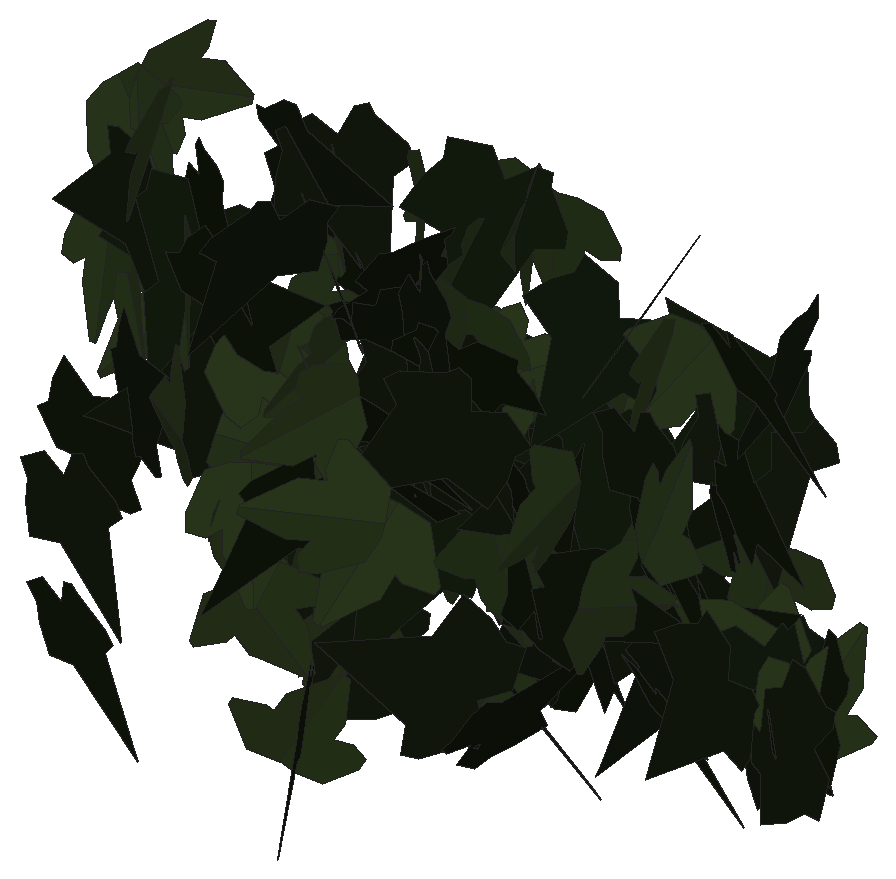
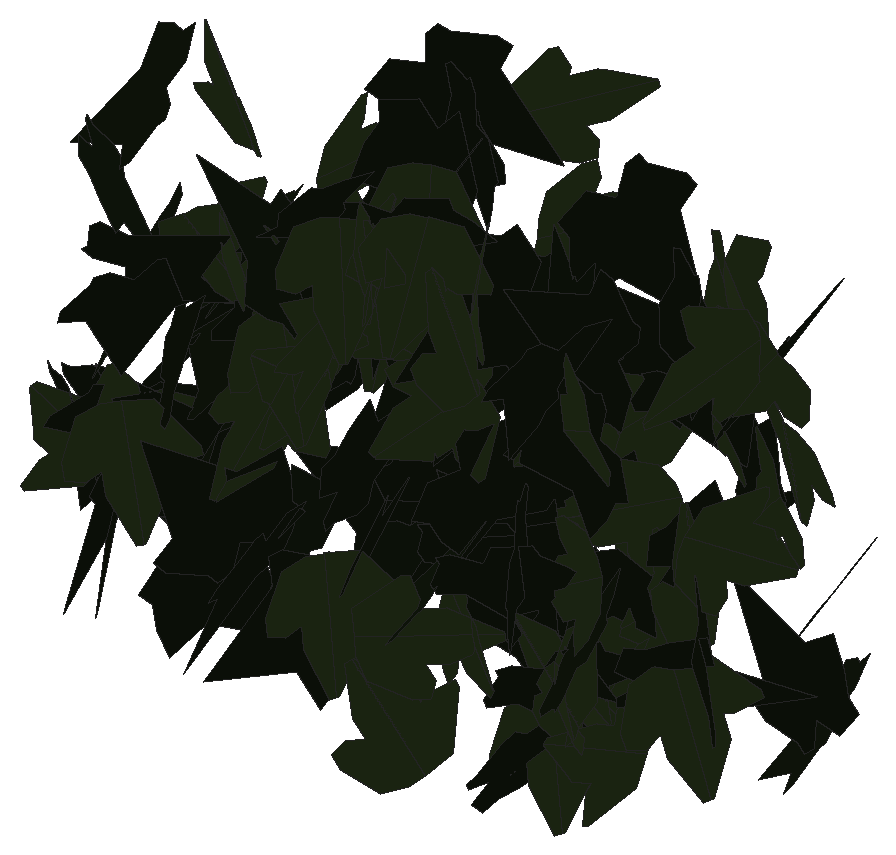
# SketchUp Ruby script. Lengths in inches.
U = 1.inch
M = Sketchup.active_model
def pt(a) = Geom::Point3d.new(a.map { |v| v * U })
def face(e, loops, mat)
  f = e.add_face(loops[0].map { |a| pt(a) })
  loops[1..].each { |l| e.add_face(l.map { |a| pt(a) }).erase! }
  f.material = f.back_material = mat if mat
  f
end
# faces: each face lists its corners as indices into pts; further lists are holes
def faces(e, pts, list, mat = nil) = list.each { |f| face(e, (f[0].is_a?(Array) ? f : [f]).map { |l| l.map { |i| pts[i] } }, mat) }
# xy, xz, yz: faces in a plane at the given z, y or x. An outline is a flat list of corners, or four numbers for a rectangle; further outlines are holes
def ring(l) = l.size == 4 ? [[l[0], l[1]], [l[2], l[1]], [l[2], l[3]], [l[0], l[3]]] : l.each_slice(2).to_a
def flat(e, list, mat, &to3) = list.each { |f| face(e, (f[0].is_a?(Array) ? f : [f]).map { |l| ring(l).map { |u, v| to3.(u, v) } }, mat) }
def xy(e, z, list, mat = nil) = flat(e, list, mat) { |x, y| [x, y, z] }
def xz(e, y, list, mat = nil) = flat(e, list, mat) { |x, z| [x, y, z] }
def yz(e, x, list, mat = nil) = flat(e, list, mat) { |y, z| [x, y, z] }
def lines(e, pts, list) = list.each { |a, b| e.add_line(pt(pts[a]), pt(pts[b])) }
# prism: a flat outline (further loops are holes) pulled along v
def prism(e, loops, v, mat = nil)
  f = face(e, loops, mat); d = Geom::Vector3d.new(v.map { |x| x * U })
  f.pushpull(f.normal.samedirection?(d) ? d.length : -d.length)
end
def box(e, o, s, mat = nil) = prism(e, [[o, [o[0] + s[0], o[1], o[2]], [o[0] + s[0], o[1] + s[1], o[2]], [o[0], o[1] + s[1], o[2]]]], [0, 0, s[2]], mat)
def at(x, y, z, deg = 0) = Geom::Transformation.translation(pt([x, y, z])) * Geom::Transformation.rotation(ORIGIN, Z_AXIS, deg.degrees)
def axes(o, x, y, z) = Geom::Transformation.new([*x, 0, *y, 0, *z, 0, *pt(o).to_a, 1])
def part(name) = M.definitions.add(name)
# library, detail: a bought-in or finely detailed component or shape, given as its bounding box
def library(name, o, s) = part(name).tap { |d| box(d.entities, o, s) }
def detail(e, o, s) = box(e.add_group.entities, o, s)
def put(e, d, t, mat = nil) = e.add_instance(d, t).tap { |i| i.material = mat if mat }
def group(e, t, mat = nil) = e.add_group.tap { |g| g.transformation = t; g.material = mat if mat }.entities
root = M.entities
M.materials.add("efeu1").color = [18, 25, 13]
M.materials.add("efeu2").color = [43, 57, 29]
c1 = part("ivyleaf_10")
p = [[0,0.5,-0.03],[-0.0625,2.02,-0.43],[-0.19,2.01,-0.46],[-0.54,1.05,-0.29],[-0.52,0.625,-0.18],[-0.83,0.76,-0.28],
  [-1.16,0.64,-0.33],[-1.15,0.33,-0.24],[-0.77,-0.39,0.02],[-0.3,-0.51,0.16],[0.04,-0.48,0.23],[-0.02,2.01,-0.4375],
  [-0.06,2.01,-0.43],[0.04,-0.49,0.23],[0.67,-0.49,0.14],[1.38,0.36,-0.2],[1.375,0.51,-0.24],[0.81,0.65,-0.19],
  [0.62,0.59,-0.15],[0.6,1.09,-0.28],[0.5,1.23,-0.31]]
faces(c1.entities,p,[[0,1,2,3,4,5,6,7,8,9,10],[11,12,0,13,14,15,16,17,18,19,20]],"efeu2")
c2 = part("ivyleaf_9")
p = [[1.54,2.16,1.25],[1.36,2.04,1.19],[-0.21,0.99,0.68],[-0.71,1.11,0.82],[-0.85,0.86,0.67],[-0.8,0.17,0.21],
  [-0.9,-0.01,0.1],[-0.67,-0.16,-0.02],[-0.08,-0.08,-0.05],[-0.03,-0.6,-0.4],[0.65,-0.88,-0.66],[0.83,-0.6,-0.49],
  [1.29,-0.42,-0.43],[1.8125,-0.07,-0.26],[1.21,0.44,0.15]]
faces(c2.entities,p,[[0,1,2,3,4,5,6,7,8,9,10,11,12,13,14]],"efeu1")
put(root,c1,axes([36.13,218.96,206],[0.03436,0.12962,0.48168],[-0.23138,-0.4236,0.13049],[0.44191,-0.23187,0.03087]))
put(root,c2,axes([36.56,219.97,206.74],[0.03192,0.04835,-0.49663],[-0.22074,-0.44493,-0.0575],[-0.4475,0.22293,-0.00706]))
put(root,c1,axes([33.57,219.77,205.62],[-0.07264,0.05256,0.49189],[-0.44926,0.20113,-0.08784],[-0.2071,-0.45474,0.01801]))
put(root,c1,axes([34.77,220.44,205.97],[0.05245,0.07368,-0.49175],[-0.23204,-0.43371,-0.08974],[-0.43978,0.23763,-0.0113]))
put(root,c1,axes([37.06,220.62,205.8],[0.00219,-0.06715,0.49546],[0.17752,-0.46309,-0.06355],[0.46742,0.17618,0.02181]))
put(root,c1,axes([38.2,220.55,205.84],[0.42828,-0.22801,-0.12078],[0.1093,-0.05169,0.48516],[-0.23373,-0.44197,0.00557]))
put(root,c2,axes([34.06,220.9,202.68],[-0.17034,0.06798,-0.46515],[0.42163,-0.19668,-0.18315],[-0.20787,-0.45464,0.00968]))
put(root,c1,axes([36.4,220.68,204.99],[-0.4722,-0.15824,-0.04459],[0.04241,0.01377,-0.49801],[0.15883,-0.4741,0.00042]))
put(root,c2,axes([35.78,221.01,203.21],[-0.10954,0.01094,0.48773],[-0.46596,-0.1504,-0.10128],[0.14449,-0.47672,0.04314]))
put(root,c2,axes([35.31,220.92,207],[-0.10485,-0.01012,-0.48878],[0.48868,0.01233,-0.10508],[0.01418,-0.49975,0.0073]))
put(root,c2,axes([31.36,220.94,202.57],[0.31223,-0.39042,0.00924],[0.00571,-0.00726,-0.49991],[0.39049,0.31228,-0.00007]))
put(root,c2,axes([31.34,220.98,203.79],[0.22591,-0.44423,-0.04032],[-0.01843,0.03586,-0.49837],[0.44568,0.22666,-0.00017]))
put(root,c2,axes([35.81,220.82,206.7],[0.32221,0.24175,-0.29621],[-0.25215,-0.15683,-0.40227],[-0.28741,0.40861,0.02085]))
put(root,c2,axes([31.91,221.1875,204.64],[-0.01304,0.05381,0.49693],[0.20362,-0.45341,0.05444],[0.45648,0.20378,-0.01008]))
put(root,c1,axes([33.97,221.22,205.26],[-0.19015,0.04104,0.46061],[0.39636,-0.24207,0.1852],[0.2382,0.43557,0.05952]))
put(root,c2,axes([36.1875,220.85,205.84],[0.36139,0.02639,-0.34453],[-0.34482,-0.00452,-0.36205],[-0.02222,0.49928,0.01493]))
put(root,c2,axes([33.5,221.18,207],[-0.07327,0.294,-0.39774],[0.07631,-0.39055,-0.30274],[-0.48868,-0.10507,0.01237]))
put(root,c2,axes([35.53,221.17,206.36],[0.22238,-0.44602,-0.04013],[-0.01749,0.03612,-0.49839],[0.44748,0.22307,0.00047]))
put(root,c2,axes([38.2,221.48,204],[-0.10345,-0.34738,0.34442],[-0.07749,-0.33595,-0.36212],[0.483,-0.1283,0.01567]))
put(root,c1,axes([37.34,220.77,204.79],[-0.0685,-0.18944,-0.45762],[0.15436,0.4308,-0.20145],[0.47062,-0.16887,-0.00053]))
put(root,c2,axes([36.76,220.89,204.67],[0.08424,0.10488,-0.48156],[0.2523,0.4105,0.13354],[0.42338,-0.26549,0.01623]))
put(root,c2,axes([33.72,221.38,204.41],[-0.0777,0.15834,-0.46786],[0.10826,-0.45663,-0.17252],[-0.48192,-0.12811,0.03667]))
put(root,c1,axes([33.7,221.15,201.92],[-0.38162,-0.23646,0.22012],[0.19271,0.10681,0.44884],[-0.25929,0.42741,0.00962]))
put(root,c2,axes([36.6,220.88,204.49],[-0.05901,-0.1327,0.47844],[0.18507,0.44121,0.1452],[-0.46072,0.19423,-0.00296]))
put(root,c2,axes([35.93,220.92,202.88],[0.09882,0.47935,-0.10227],[0.01039,0.10226,0.48932],[0.49003,-0.09883,0.01025]))
put(root,c2,axes([34.29,221.09,205.55],[0.48925,-0.04896,0.09077],[0.09039,-0.00828,-0.49169],[0.04965,0.49753,0.00075]))
put(root,c2,axes([32.57,221.49,205.73],[0.07605,-0.04883,0.49176],[0.40737,-0.27548,-0.09035],[0.27976,0.4144,-0.00211]))
put(root,c1,axes([32.96,221.45,204.05],[0.48071,0.09544,0.09905],[0.09726,0.01874,-0.49009],[-0.09726,0.49045,-0.00055]))
put(root,c1,axes([33.56,221.89,205.39],[-0.00246,0.05499,-0.49696],[-0.07722,-0.49105,-0.05396],[-0.49399,0.07649,0.01091]))
put(root,c1,axes([33.02,221.43,203.05],[-0.34348,-0.28151,-0.22972],[0.1933,0.12609,-0.44355],[0.30766,-0.39351,0.02222]))
put(root,c2,axes([36.2,221.96,204.95],[0.10369,-0.33735,-0.35418],[0.12042,-0.3333,0.35272],[-0.47408,-0.15844,0.01213]))
put(root,c1,axes([35.36,221.55,206.59],[-0.49125,-0.00203,0.09309],[-0.09307,-0.00365,-0.49125],[0.00268,-0.49998,0.00321]))
put(root,c1,axes([34.2,221.75,204],[0.37428,0.22882,-0.23991],[-0.20542,-0.12395,-0.43868],[-0.26023,0.42694,0.00122]))
put(root,c2,axes([31.44,222.02,206.17],[0.18723,-0.39573,-0.24155],[0.12156,-0.20949,0.43742],[-0.4474,-0.22252,0.01776]))
put(root,c1,axes([31.81,221.9,205.76],[0.26744,-0.12228,0.40438],[0.35526,-0.19389,-0.29359],[0.22861,0.44436,-0.01682]))
put(root,c1,axes([31.625,221.89,207.18],[0.20755,-0.42845,0.15281],[0.07003,-0.13586,-0.47606],[0.44946,0.21902,0.00361]))
put(root,c2,axes([32.1,221.89,206.625],[0.00328,-0.02406,-0.49941],[0.49999,0.00004,0.00328],[-0.00012,-0.49942,0.02406]))
put(root,c1,axes([32.8125,221.62,204.46],[-0.12623,-0.0831,-0.47661],[0.45921,0.13448,-0.14507],[0.1523,-0.47435,0.04237]))
put(root,c1,axes([31.04,221.88,205.83],[0.44069,-0.19571,0.13223],[0.12062,-0.05418,-0.4822],[0.20307,0.4569,-0.00054]))
put(root,c2,axes([32.1,222.16,204.37],[-0.12736,-0.14326,0.4618],[-0.3104,-0.34192,-0.19168],[0.37071,-0.33551,-0.00184]))
put(root,c1,axes([32.86,221.62,205.34],[0.21763,0.2164,0.39472],[0.27686,0.28135,-0.3069],[-0.35494,0.35215,0.00263]))
put(root,c2,axes([32,222.05,206.13],[-0.34557,-0.3466,-0.1022],[0.07348,0.07106,-0.48944],[0.35381,-0.35329,0.00182]))
put(root,c2,axes([36.875,221.94,205.74],[0.26153,-0.4258,-0.01719],[-0.00564,0.01671,-0.49969],[0.42611,0.26156,0.00394]))
put(root,c2,axes([35.08,221.7,205.24],[0.47595,-0.04793,-0.14552],[-0.14421,0.02023,-0.47832],[0.05174,0.49729,0.00544]))
put(root,c2,axes([33.3125,222.19,205.99],[-0.00947,-0.13019,0.48266],[0.15544,-0.45958,-0.12092],[0.47513,0.14776,0.04918]))
put(root,c2,axes([38.84,221.85,203.42],[-0.24425,-0.04393,-0.43406],[-0.4142,-0.13291,0.24652],[-0.13704,0.48001,0.02854]))
put(root,c2,axes([37.92,221.98,206.93],[0.37108,-0.3283,0.06723],[0.05323,-0.04129,-0.49544],[0.33086,0.37485,0.0043]))
put(root,c2,axes([37.02,222.07,203.15],[0.30507,-0.33252,0.21532],[0.15295,-0.15184,-0.45117],[0.36543,0.34114,0.00907]))
put(root,c2,axes([36.97,222.16,204.73],[0.21579,-0.37594,0.2492],[0.1183,-0.21941,-0.43343],[0.43525,0.24602,-0.00575]))
put(root,c2,axes([37.08,222.26,203.99],[0.10126,-0.3108,0.37835],[0.13148,-0.35491,-0.32673],[0.47165,0.16566,0.00986]))
put(root,c1,axes([32.62,221.61,203.56],[0.06943,-0.11964,0.48049],[-0.21838,0.42805,0.13814],[-0.4444,-0.22904,0.00718]))
put(root,c2,axes([35.29,221.95,202.93],[0.43804,-0.23577,0.0503],[0.04428,-0.02387,-0.49746],[0.23698,0.44028,-0.00003]))
put(root,c2,axes([30.66,222.07,203.35],[-0.07305,0.05429,0.49165],[0.35331,-0.34209,0.09028],[0.34617,0.36059,0.01162]))
put(root,c1,axes([30.92,222.2,205.41],[0.2844,-0.11415,0.39508],[0.37324,-0.13003,-0.30624],[0.17266,0.46911,0.01125]))
put(root,c2,axes([34.3,222.28,203.88],[-0.42939,-0.24211,-0.08368],[0.07392,0.03928,-0.49294],[0.24527,-0.4357,0.00206]))
put(root,c2,axes([36.1875,222.49,206.41],[-0.19617,-0.4125,0.20338],[-0.07115,-0.19123,-0.45647],[0.45437,-0.20803,0.01633]))
put(root,c2,axes([35.92,222.45,203.3125],[0.08722,-0.28655,0.40036],[0.14023,-0.37529,-0.29916],[0.47194,0.16447,0.0149]))
put(root,c2,axes([35.4,222.56,203.15],[-0.04846,-0.18391,0.46242],[-0.05841,-0.45929,-0.18878],[0.49421,-0.07231,0.02303]))
put(root,c2,axes([36.28,222.35,205.5],[-0.24472,-0.41052,-0.14694],[0.07222,0.12801,-0.47791],[0.43,-0.25513,-0.00335]))
put(root,c2,axes([34.03,221.95,206.03],[0.37988,0.3247,-0.01616],[-0.01291,-0.00978,-0.49974],[-0.32485,0.3801,0.00095]))
put(root,c1,axes([35.16,222.17,205.64],[0.24935,-0.10655,-0.42009],[0.43203,0.02274,0.25067],[-0.03431,-0.48799,0.1034]))
put(root,c1,axes([31.39,222.58,204.96],[-0.12276,-0.1985,0.44218],[-0.04185,-0.4501,-0.21367],[0.48289,-0.08947,0.0939]))
put(root,c2,axes([38.05,222.25,203.9],[-0.09692,-0.38236,-0.30726],[0.0799,0.29671,-0.39444],[0.48397,-0.12555,0.00359]))
put(root,c1,axes([33.375,222.29,202.42],[-0.3226,-0.3795,0.0437],[-0.02704,-0.03436,-0.49808],[0.38105,-0.32373,0.00165]))
put(root,c1,axes([30.93,222.31,206.81],[0.37286,0.01551,0.33277],[0.33178,0.02757,-0.37304],[-0.02992,0.499,0.01027]))
put(root,c1,axes([37.98,222.38,203.72],[0.19088,0.12287,0.4455],[-0.38769,-0.21976,0.22672],[0.25152,-0.43198,0.01138]))
put(root,c2,axes([37.75,222.13,205.64],[0.35868,-0.1875,-0.29358],[-0.24565,0.16263,-0.40399],[0.24699,0.43404,0.02455]))
put(root,c1,axes([33.11,221.96,205.58],[-0.03813,-0.16625,-0.47001],[0.17888,0.43543,-0.16853],[0.46535,-0.181,0.02627]))
put(root,c1,axes([34.59,222.68,206.34],[-0.00063,0.01045,-0.49989],[-0.07525,-0.4942,-0.01024],[-0.49431,0.07522,0.00219]))
put(root,c2,axes([33.98,221.92,206.22],[0.24782,0.29857,0.31534],[0.18836,0.25325,-0.3878],[-0.39129,0.311,0.01304]))
put(root,c2,axes([33.39,222.49,203.29],[-0.42756,-0.13134,-0.22349],[0.21282,0.06826,-0.44727],[0.148,-0.47759,-0.00247]))
put(root,c2,axes([33.5,222.4375,203.88],[0.38893,0.05681,-0.30904],[0.30444,0.05359,0.39299],[0.07778,-0.49386,0.0071]))
put(root,c2,axes([37.03,222.39,203.53],[0.01008,-0.04979,0.49741],[0.45453,-0.20618,-0.02985],[0.20808,0.45278,0.04111]))
put(root,c2,axes([38.8,222.2,203.57],[-0.17873,0.00667,-0.46692],[-0.46607,0.0284,0.17881],[0.02891,0.49915,-0.00393]))
put(root,c1,axes([36.6,222.62,206.26],[0.19052,-0.39176,0.2454],[0.11495,-0.21694,-0.43557],[0.44776,0.22239,0.0074]))
put(root,c2,axes([38.11,222.25,203.4],[0.21889,-0.05425,-0.44626],[-0.41837,0.15703,-0.2243],[0.16449,0.47159,0.02335]))
put(root,c2,axes([32.75,222.51,204.36],[-0.24147,-0.16728,-0.40461],[0.32699,0.23837,-0.2937],[0.29115,-0.40644,-0.00572]))
put(root,c2,axes([38.03,222.28,203.38],[0.18523,-0.18948,-0.42401],[-0.2968,0.30281,-0.26498],[0.35721,0.34986,-0.0003]))
put(root,c1,axes([38.43,222.24,203.32],[0.24952,0.29387,-0.3184],[0.2064,0.24244,0.38552],[0.38097,-0.32382,-0.00032]))
put(root,c1,axes([31.53,222.64,204.21],[0.08658,-0.47022,-0.14629],[0.02485,-0.14417,0.47812],[-0.49182,-0.09007,-0.00159]))
put(root,c2,axes([33.85,222.86,204.96],[-0.03043,-0.06052,-0.49539],[0.041,-0.49494,0.05794],[-0.49739,-0.03709,0.03509]))
put(root,c1,axes([32.75,222.79,203.29],[0.15857,-0.34946,0.32052],[0.14693,-0.28512,-0.38356],[0.45085,0.21583,0.01227]))
put(root,c2,axes([33.01,222.8,203.26],[-0.27705,-0.41282,-0.05317],[0.02882,0.04469,-0.49716],[0.41523,-0.27854,-0.00097]))
put(root,c2,axes([34.73,222.76,207.13],[-0.3411,-0.33574,-0.14468],[0.09653,0.10815,-0.47853],[0.35261,-0.35438,-0.00896]))
put(root,c1,axes([33.73,222.86,206.61],[0.02856,-0.07796,0.49306],[0.39049,-0.30416,-0.07071],[0.31097,0.38911,0.04351]))
put(root,c2,axes([33.5,222.9,202.08],[-0.02183,-0.47668,-0.14935],[0.02422,-0.15032,0.47625],[-0.49894,0.01356,0.02965]))
put(root,c1,axes([32.51,222.29,202.4],[0.08247,0.17878,-0.4596],[0.20057,0.41354,0.19686],[0.45052,-0.21684,-0.00351]))
put(root,c2,axes([36.11,222.47,205.97],[-0.0418,0.48767,0.10213],[0.00163,-0.10236,0.48941],[0.49825,0.04124,0.00696]))
put(root,c1,axes([36.86,222.72,206.2],[0.41684,0.05033,-0.2715],[-0.27113,-0.01855,-0.4197],[-0.05232,0.49711,0.01183]))
put(root,c2,axes([38,222.77,206.6],[-0.39436,0.24912,-0.18004],[0.15441,-0.09266,-0.46645],[-0.26577,-0.4235,-0.00385]))
put(root,c1,axes([33.99,222.73,205.86],[0.08055,-0.49145,0.04465],[0.00919,0.04673,0.49773],[-0.49338,-0.07936,0.01656]))
put(root,c1,axes([35.52,222.57,205.6],[-0.02103,0.48353,0.12554],[-0.00604,0.1254,-0.48398],[-0.49952,-0.02187,0.00057]))
put(root,c1,axes([36.18,222.57,204.74],[-0.2193,-0.34691,-0.28559],[0.18295,0.22132,-0.40933],[0.41041,-0.28403,0.02986]))
put(root,c1,axes([34.77,223.1,206.67],[0.03185,-0.08691,-0.49136],[0.10014,-0.48123,0.09161],[-0.48883,-0.10425,-0.01325]))
put(root,c2,axes([32.27,222.81,206.61],[0.28532,0.00581,-0.41056],[0.39294,0.14117,0.27508],[0.11911,-0.47962,0.076]))
put(root,c1,axes([32.5,222.91,204.4],[-0.21106,0.19718,-0.40814],[0.30103,-0.27561,-0.28882],[-0.33887,-0.36764,-0.00237]))
put(root,c2,axes([36.68,223.03,203.19],[-0.04768,0.15351,-0.47346],[0.12778,-0.45591,-0.16069],[-0.48104,-0.13632,0.00424]))
put(root,c2,axes([37.31,222.67,204.6],[0.02891,-0.27433,0.41702],[-0.06636,0.4119,0.27556],[-0.49473,-0.07128,-0.01259]))
put(root,c1,axes([34.0625,222.74,205.54],[-0.35745,-0.0242,-0.34877],[0.34873,0.01064,-0.35815],[0.02475,-0.4993,0.00927]))
put(root,c2,axes([34.02,223.01,203.92],[0.19121,-0.44716,0.11615],[0.06109,-0.10013,-0.48605],[0.45794,0.20006,0.01634]))
put(root,c1,axes([34.17,222.67,203.43],[-0.12399,0.07652,0.4783],[-0.45836,0.14112,-0.1414],[-0.15664,-0.47353,0.03515]))
put(root,c1,axes([35.83,222.9,205.64],[-0.28106,-0.40745,0.07065],[-0.03971,-0.05843,-0.49498],[0.41161,-0.28385,0.00049]))
put(root,c1,axes([32.65,222.94,203.13],[-0.24422,-0.01049,0.43617],[0.43472,-0.04842,0.24224],[0.03716,0.49754,0.03277]))
put(root,c2,axes([34.92,223.25,204.61],[-0.06539,-0.11689,0.48173],[-0.21919,-0.429,-0.13384],[0.44461,-0.22869,0.00486]))
put(root,c2,axes([37.56,222.85,205.69],[-0.43655,-0.19138,-0.151],[-0.13876,-0.05956,0.47665],[-0.20043,0.45807,-0.00111]))
put(root,c2,axes([37.41,222.98,205.63],[-0.11378,-0.44998,-0.18594],[0.03919,0.18186,-0.4641],[0.4853,-0.12019,-0.00612]))
put(root,c2,axes([33.43,223.1,204.28],[-0.38114,-0.3172,-0.06417],[0.05262,0.03709,-0.49584],[0.31932,-0.38472,0.00511]))
put(root,c1,axes([35.37,222.89,203.33],[-0.31236,-0.389,0.03335],[-0.02,-0.02672,-0.49889],[0.38992,-0.31299,0.00113]))
put(root,c1,axes([34.53,222.82,201.94],[-0.17496,-0.42433,0.19833],[0.08177,0.18079,0.45894],[-0.4612,0.19303,0.00613]))
put(root,c1,axes([34.39,222.83,206.98],[-0.3736,-0.31166,-0.11529],[0.0888,0.07353,-0.48653],[0.32021,-0.38401,0.00041]))
put(root,c2,axes([31.61,223.15,203.77],[-0.33629,-0.08683,0.35968],[-0.34148,-0.11432,-0.34687],[0.14247,-0.47895,0.01759]))
put(root,c1,axes([31.13,222.55,206.94],[0.07649,0.16146,0.46699],[0.03822,0.4692,-0.16849],[-0.49263,0.06147,0.05944]))
put(root,c2,axes([32.31,223.28,203.78],[0.07836,-0.33562,0.36224],[0.09122,-0.35062,-0.34459],[0.48532,0.12009,0.00628]))
put(root,c1,axes([35.74,222.61,205.0625],[0.10809,0.28284,-0.39789],[0.11848,0.38014,0.30241],[0.47358,-0.15966,0.01515]))
put(root,c2,axes([35.61,222.62,202.93],[-0.05363,0.21104,-0.4501],[-0.15407,0.42336,0.21686],[0.47264,0.16195,0.01962]))
put(root,c2,axes([36.03,222.95,203.5],[0.24131,-0.33341,-0.28391],[-0.14587,0.24445,-0.41106],[0.41291,0.28121,0.02071]))
put(root,c2,axes([32.96,223.3,204.68],[-0.0786,0.05318,-0.49091],[0.44599,-0.20571,-0.09369],[-0.21194,-0.45261,-0.0151]))
put(root,c2,axes([32.22,223.11,205.95],[0.02646,0.0007,-0.4993],[0.47872,0.14202,0.02557],[0.14186,-0.4794,0.00684]))
put(root,c1,axes([37.45,223.1,204.2],[-0.43621,-0.209,0.12667],[-0.10673,-0.07022,-0.4834],[0.21985,-0.44877,0.01664]))
put(root,c1,axes([31.28,223.16,203.83],[-0.34399,-0.33135,0.14791],[-0.10686,-0.10226,-0.47762],[0.34677,-0.36021,-0.00047]))
put(root,c2,axes([31.24,222.77,203.84],[0.02798,0.00262,0.49921],[-0.02736,0.49925,-0.00108],[-0.49847,-0.02726,0.02809]))
put(root,c2,axes([32.63,223.13,206.67],[0.0401,-0.4405,-0.23314],[-0.02399,0.23191,-0.44231],[0.49781,0.04666,-0.00254]))
put(root,c1,axes([32.1875,223.27,206.13],[0.21973,-0.05656,0.44555],[0.4235,-0.13908,-0.22651],[0.14956,0.47693,-0.01321]))
put(root,c1,axes([34.35,223.36,203.34],[0.01322,0.05362,0.49694],[-0.31332,-0.38643,0.05003],[0.38943,-0.31272,0.02339]))
put(root,c1,axes([35.08,223.12,206.85],[-0.47873,-0.09428,0.10922],[-0.1047,-0.03346,-0.48777],[0.09928,-0.48989,0.0123]))
put(root,c2,axes([36.3125,222.95,203.49],[-0.13387,-0.12084,0.46634],[0.42534,0.19762,0.17331],[-0.2262,0.44311,0.04988]))
